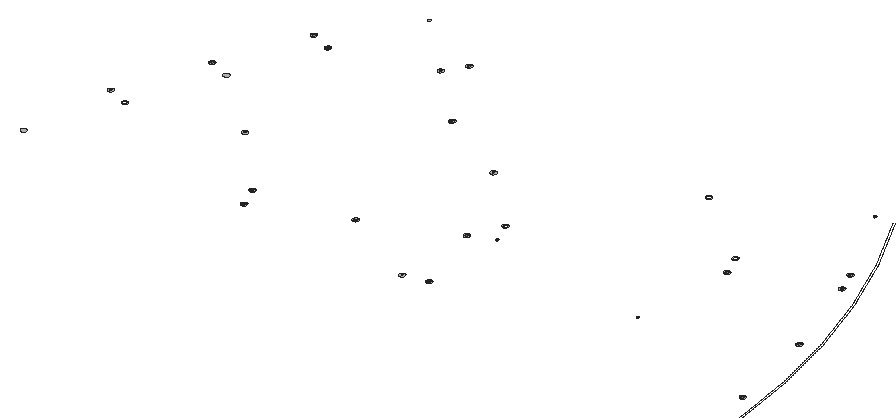
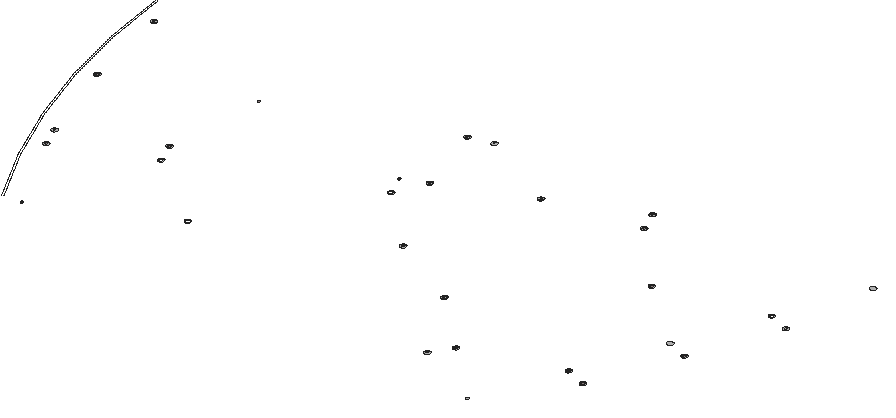
# SketchUp Ruby script. Lengths in inches.
U = 1.inch
M = Sketchup.active_model
def pt(a) = Geom::Point3d.new(a.map { |v| v * U })
def face(e, loops, mat)
  f = e.add_face(loops[0].map { |a| pt(a) })
  loops[1..].each { |l| e.add_face(l.map { |a| pt(a) }).erase! }
  f.material = f.back_material = mat if mat
  f
end
# faces: each face lists its corners as indices into pts; further lists are holes
def faces(e, pts, list, mat = nil) = list.each { |f| face(e, (f[0].is_a?(Array) ? f : [f]).map { |l| l.map { |i| pts[i] } }, mat) }
# xy, xz, yz: faces in a plane at the given z, y or x. An outline is a flat list of corners, or four numbers for a rectangle; further outlines are holes
def ring(l) = l.size == 4 ? [[l[0], l[1]], [l[2], l[1]], [l[2], l[3]], [l[0], l[3]]] : l.each_slice(2).to_a
def flat(e, list, mat, &to3) = list.each { |f| face(e, (f[0].is_a?(Array) ? f : [f]).map { |l| ring(l).map { |u, v| to3.(u, v) } }, mat) }
def xy(e, z, list, mat = nil) = flat(e, list, mat) { |x, y| [x, y, z] }
def xz(e, y, list, mat = nil) = flat(e, list, mat) { |x, z| [x, y, z] }
def yz(e, x, list, mat = nil) = flat(e, list, mat) { |y, z| [x, y, z] }
def lines(e, pts, list) = list.each { |a, b| e.add_line(pt(pts[a]), pt(pts[b])) }
# prism: a flat outline (further loops are holes) pulled along v
def prism(e, loops, v, mat = nil)
  f = face(e, loops, mat); d = Geom::Vector3d.new(v.map { |x| x * U })
  f.pushpull(f.normal.samedirection?(d) ? d.length : -d.length)
end
def box(e, o, s, mat = nil) = prism(e, [[o, [o[0] + s[0], o[1], o[2]], [o[0] + s[0], o[1] + s[1], o[2]], [o[0], o[1] + s[1], o[2]]]], [0, 0, s[2]], mat)
def at(x, y, z, deg = 0) = Geom::Transformation.translation(pt([x, y, z])) * Geom::Transformation.rotation(ORIGIN, Z_AXIS, deg.degrees)
def axes(o, x, y, z) = Geom::Transformation.new([*x, 0, *y, 0, *z, 0, *pt(o).to_a, 1])
def part(name) = M.definitions.add(name)
# library, detail: a bought-in or finely detailed component or shape, given as its bounding box
def library(name, o, s) = part(name).tap { |d| box(d.entities, o, s) }
def detail(e, o, s) = box(e.add_group.entities, o, s)
def put(e, d, t, mat = nil) = e.add_instance(d, t).tap { |i| i.material = mat if mat }
def group(e, t, mat = nil) = e.add_group.tap { |g| g.transformation = t; g.material = mat if mat }.entities
root = M.entities
M.materials.add("[Asphalt_Stamped_Brick]").color = [149, 133, 134]
M.materials.add("[Metal_Steel_Textured_White]").color = [191, 191, 191]
xy(root,3.625,[[165.183,166.325,165.178,166.327,165.174,166.33,165.171,166.335,165.169,166.339,165.168,166.345,165.169,166.35,165.171,166.355,165.174,166.359,165.178,166.362,165.183,166.364,165.188,166.365,165.193,166.364,165.198,166.362,165.202,166.359,165.205,166.355,165.207,166.35,165.208,166.345,165.207,166.339,165.205,166.335,165.202,166.33,165.198,166.327,165.193,166.325],[158.582,166.555,158.577,166.556,158.572,166.558,158.568,166.561,158.564,166.565,158.5625,166.57,158.562,166.575,158.5625,166.581,158.564,166.585,158.568,166.59,158.572,166.593,158.577,166.595,158.587,166.595,158.592,166.593,158.596,166.59,158.599,166.585,158.601,166.581,158.602,166.575,158.601,166.57,158.599,166.565,158.596,166.561,158.592,166.558,158.587,166.556],[175.826,166.647,175.821,166.648,175.816,166.65,175.812,166.653,175.809,166.657,175.807,166.662,175.806,166.667,175.807,166.672,175.809,166.677,175.812,166.681,175.816,166.685,175.821,166.687,175.831,166.687,175.836,166.685,175.84,166.681,175.843,166.677,175.845,166.672,175.846,166.667,175.845,166.662,175.843,166.657,175.84,166.653,175.836,166.65,175.831,166.648],[158.276,167.293,158.271,167.294,158.266,167.296,158.262,167.299,158.259,167.303,158.257,167.308,158.256,167.313,158.257,167.318,158.259,167.323,158.262,167.327,158.266,167.33,158.271,167.332,158.276,167.333,158.281,167.332,158.286,167.33,158.29,167.327,158.294,167.323,158.296,167.318,158.296,167.308,158.294,167.303,158.29,167.299,158.286,167.296,158.281,167.294],[170.838,168.324,170.833,168.326,170.829,168.329,170.826,168.334,170.824,168.338,170.823,168.344,170.824,168.349,170.826,168.354,170.829,168.358,170.833,168.361,170.838,168.363,170.843,168.364,170.849,168.363,170.853,168.361,170.858,168.358,170.861,168.354,170.863,168.349,170.863,168.338,170.861,168.334,170.858,168.329,170.853,168.326,170.849,168.324],
  [164.389,168.961,164.384,168.962,164.379,168.964,164.375,168.967,164.372,168.971,164.37,168.976,164.369,168.981,164.37,168.986,164.372,168.991,164.375,168.995,164.379,168.998,164.384,169,164.389,169.001,164.395,169,164.399,168.998,164.403,168.995,164.407,168.991,164.409,168.986,164.409,168.976,164.407,168.971,164.403,168.967,164.399,168.964,164.395,168.962],[165.183,169.292,165.178,169.294,165.174,169.298,165.171,169.302,165.169,169.307,165.168,169.312,165.169,169.317,165.171,169.322,165.174,169.326,165.178,169.329,165.183,169.331,165.188,169.332,165.193,169.331,165.198,169.329,165.202,169.326,165.205,169.322,165.207,169.317,165.208,169.312,165.207,169.307,165.205,169.302,165.202,169.298,165.198,169.294,165.193,169.292],[156.122,169.662,156.117,169.663,156.112,169.665,156.108,169.668,156.105,169.672,156.103,169.677,156.102,169.682,156.103,169.687,156.105,169.692,156.108,169.696,156.112,169.699,156.117,169.701,156.122,169.702,156.128,169.701,156.132,169.699,156.136,169.696,156.14,169.692,156.142,169.687,156.142,169.677,156.14,169.672,156.136,169.668,156.132,169.665,156.128,169.663],[175.208,169.885,175.202,169.886,175.198,169.888,175.193,169.891,175.19,169.895,175.188,169.9,175.1875,169.905,175.188,169.91,175.19,169.915,175.193,169.919,175.198,169.922,175.202,169.924,175.208,169.925,175.213,169.924,175.218,169.922,175.222,169.919,175.225,169.915,175.227,169.91,175.227,169.9,175.225,169.895,175.222,169.891,175.218,169.888,175.213,169.886],[171.188,171.777,171.183,171.778,171.178,171.78,171.174,171.783,171.17,171.787,171.168,171.792,171.168,171.802,171.17,171.807,171.174,171.811,171.178,171.814,171.183,171.816,171.188,171.817,171.193,171.816,171.198,171.814,171.202,171.811,171.205,171.807,171.207,171.802,171.208,171.797,171.207,171.792,171.205,171.787,171.202,171.783,171.198,171.78,171.193,171.778],
  [153.016,172.121,153.011,172.122,153.006,172.124,153.002,172.127,152.999,172.131,152.997,172.136,152.996,172.141,152.997,172.146,152.999,172.151,153.002,172.155,153.006,172.159,153.011,172.161,153.021,172.161,153.026,172.159,153.03,172.155,153.033,172.151,153.035,172.146,153.036,172.141,153.035,172.136,153.033,172.131,153.03,172.127,153.026,172.124,153.021,172.122],[162.779,172.128,162.774,172.13,162.77,172.133,162.767,172.138,162.765,172.142,162.764,172.147,162.765,172.153,162.767,172.157,162.77,172.162,162.774,172.165,162.779,172.167,162.789,172.167,162.794,172.165,162.798,172.162,162.801,172.157,162.803,172.153,162.804,172.147,162.803,172.142,162.801,172.138,162.798,172.133,162.794,172.13,162.789,172.128],[174.183,173.02,174.178,173.022,174.174,173.025,174.17,173.03,174.168,173.034,174.168,173.045,174.17,173.05,174.174,173.054,174.178,173.057,174.183,173.059,174.1875,173.06,174.193,173.059,174.198,173.057,174.202,173.054,174.205,173.05,174.207,173.045,174.208,173.04,174.207,173.034,174.205,173.03,174.202,173.025,174.198,173.022,174.193,173.02],[173.882,173.757,173.877,173.758,173.872,173.76,173.868,173.763,173.865,173.767,173.863,173.772,173.862,173.777,173.863,173.782,173.865,173.787,173.868,173.791,173.872,173.795,173.877,173.797,173.887,173.797,173.892,173.795,173.896,173.791,173.899,173.787,173.901,173.782,173.902,173.777,173.901,173.772,173.899,173.767,173.896,173.763,173.892,173.76,173.887,173.758],[154.951,174.72,154.946,174.722,154.942,174.725,154.939,174.73,154.937,174.734,154.936,174.74,154.937,174.745,154.939,174.75,154.942,174.754,154.946,174.757,154.951,174.759,154.956,174.76,154.962,174.759,154.966,174.757,154.97,174.754,154.974,174.75,154.976,174.745,154.976,174.734,154.974,174.73,154.97,174.725,154.966,174.722,154.962,174.72],
  [154.219,175.025,154.214,175.026,154.209,175.028,154.205,175.031,154.201,175.035,154.199,175.04,154.199,175.05,154.201,175.055,154.205,175.059,154.209,175.0625,154.214,175.064,154.219,175.065,154.224,175.064,154.229,175.0625,154.233,175.059,154.236,175.055,154.238,175.05,154.239,175.045,154.238,175.04,154.236,175.035,154.233,175.031,154.229,175.028,154.224,175.026],[158.583,176.324,158.578,176.326,158.574,176.33,158.571,176.334,158.569,176.339,158.568,176.344,158.569,176.349,158.571,176.354,158.574,176.358,158.578,176.361,158.583,176.363,158.588,176.364,158.593,176.363,158.598,176.361,158.602,176.358,158.605,176.354,158.607,176.349,158.608,176.344,158.607,176.339,158.605,176.334,158.602,176.33,158.598,176.326,158.593,176.324],[172.387,176.695,172.382,176.696,172.377,176.698,172.373,176.701,172.37,176.705,172.368,176.71,172.367,176.715,172.368,176.72,172.37,176.725,172.373,176.729,172.377,176.732,172.382,176.734,172.387,176.735,172.392,176.734,172.397,176.732,172.401,176.729,172.404,176.725,172.406,176.72,172.407,176.715,172.406,176.71,172.404,176.705,172.401,176.701,172.397,176.698,172.392,176.696]],"[Asphalt_Stamped_Brick]")
xy(root,3.625,[[[151.348,165.94,151.325,165.943,151.304,165.952,151.286,165.966,151.272,165.984,151.263,166.005,151.26,166.028,151.263,166.051,151.272,166.072,151.286,166.09,151.304,166.104,151.325,166.113,151.348,166.116,151.371,166.113,151.392,166.104,151.41,166.09,151.424,166.072,151.433,166.051,151.436,166.028,151.433,166.005,151.424,165.984,151.41,165.966,151.392,165.952,151.371,165.943],[151.348,165.992,151.357,165.993,151.366,165.996,151.374,166.002,151.38,166.01,151.383,166.019,151.385,166.028,151.383,166.038,151.38,166.046,151.374,166.054,151.366,166.06,151.357,166.064,151.348,166.065,151.339,166.064,151.33,166.06,151.322,166.054,151.316,166.046,151.3125,166.038,151.311,166.028,151.3125,166.019,151.316,166.01,151.322,166.002,151.33,165.996,151.339,165.993]],[[164.389,166.091,164.367,166.094,164.345,166.103,164.327,166.117,164.313,166.135,164.304,166.156,164.301,166.179,164.304,166.202,164.313,166.223,164.327,166.241,164.345,166.255,164.367,166.264,164.389,166.267,164.412,166.264,164.433,166.255,164.452,166.241,164.466,166.223,164.474,166.202,164.477,166.179,164.474,166.156,164.466,166.135,164.452,166.117,164.433,166.103,164.412,166.094],[164.389,166.143,164.399,166.144,164.408,166.148,164.415,166.153,164.421,166.161,164.425,166.17,164.426,166.179,164.425,166.189,164.421,166.198,164.415,166.205,164.408,166.211,164.399,166.215,164.389,166.216,164.38,166.215,164.371,166.211,164.363,166.205,164.358,166.198,164.354,166.189,164.353,166.179,164.354,166.17,164.358,166.161,164.363,166.153,164.371,166.148,164.38,166.144]],[164.389,166.159,164.384,166.16,164.379,166.162,164.375,166.165,164.372,166.169,164.37,166.174,164.369,166.179,164.37,166.184,164.372,166.189,164.375,166.193,164.379,166.197,164.389,166.199,164.395,166.198,164.399,166.197,164.407,166.189,164.409,166.184,164.409,166.174,164.407,166.169,164.403,166.165,164.399,166.162,164.395,166.16],[[165.188,166.256,165.165,166.259,165.143,166.268,165.125,166.282,165.111,166.3,165.102,166.322,165.099,166.345,165.102,166.368,165.111,166.389,165.125,166.407,165.143,166.422,165.165,166.43,165.188,166.433,165.211,166.43,165.232,166.422,165.251,166.407,165.265,166.389,165.274,166.368,165.277,166.345,165.274,166.322,165.265,166.3,165.251,166.282,165.232,166.268,165.211,166.259],[165.188,166.257,165.211,166.26,165.232,166.268,165.25,166.282,165.264,166.301,165.273,166.322,165.276,166.345,165.273,166.367,165.264,166.389,165.25,166.407,165.232,166.421,165.211,166.43,165.188,166.433,165.165,166.43,165.144,166.421,165.126,166.407,165.112,166.389,165.103,166.367,165.1,166.345,165.103,166.322,165.112,166.301,165.126,166.282,165.144,166.268,165.165,166.26]],[[165.188,166.308,165.178,166.309,165.169,166.313,165.162,166.319,165.156,166.326,165.152,166.335,165.151,166.345,165.152,166.354,165.156,166.363,165.162,166.37,165.169,166.376,165.178,166.38,165.188,166.381,165.197,166.38,165.206,166.376,165.214,166.37,165.219,166.363,165.223,166.354,165.224,166.345,165.223,166.335,165.219,166.326,165.214,166.319,165.206,166.313,165.197,166.309],[165.183,166.325,165.193,166.325,165.198,166.327,165.202,166.33,165.205,166.335,165.207,166.339,165.208,166.345,165.207,166.35,165.205,166.355,165.202,166.359,165.198,166.362,165.193,166.364,165.188,166.365,165.183,166.364,165.178,166.362,165.174,166.359,165.171,166.355,165.169,166.35,165.168,166.345,165.169,166.339,165.171,166.335,165.174,166.33,165.178,166.327]],
  [[158.582,166.487,158.559,166.49,158.537,166.498,158.519,166.513,158.505,166.531,158.496,166.552,158.493,166.575,158.496,166.598,158.505,166.62,158.519,166.638,158.537,166.652,158.559,166.661,158.582,166.664,158.605,166.661,158.626,166.652,158.645,166.638,158.659,166.62,158.668,166.598,158.671,166.575,158.668,166.552,158.659,166.531,158.645,166.513,158.626,166.498,158.605,166.49],[158.582,166.488,158.605,166.491,158.626,166.499,158.644,166.513,158.658,166.531,158.667,166.553,158.67,166.575,158.667,166.598,158.658,166.619,158.644,166.638,158.626,166.652,158.605,166.66,158.582,166.663,158.559,166.66,158.538,166.652,158.52,166.638,158.506,166.619,158.497,166.598,158.494,166.575,158.497,166.553,158.506,166.531,158.52,166.513,158.538,166.499,158.559,166.491]],[[158.582,166.488,158.559,166.491,158.538,166.499,158.52,166.513,158.506,166.531,158.497,166.553,158.494,166.575,158.497,166.598,158.506,166.619,158.52,166.638,158.538,166.652,158.559,166.66,158.582,166.663,158.605,166.66,158.626,166.652,158.644,166.638,158.658,166.619,158.667,166.598,158.67,166.575,158.667,166.553,158.658,166.531,158.644,166.513,158.626,166.499,158.605,166.491],[158.582,166.539,158.591,166.54,158.6,166.544,158.608,166.55,158.613,166.557,158.617,166.566,158.618,166.575,158.617,166.585,158.613,166.594,158.608,166.601,158.6,166.607,158.591,166.611,158.582,166.612,158.572,166.611,158.563,166.607,158.556,166.601,158.55,166.594,158.546,166.585,158.545,166.575,158.546,166.566,158.55,166.557,158.556,166.55,158.563,166.544,158.572,166.54]],[[158.582,166.539,158.572,166.54,158.563,166.544,158.556,166.55,158.55,166.557,158.546,166.566,158.545,166.575,158.546,166.585,158.55,166.594,158.556,166.601,158.563,166.607,158.572,166.611,158.582,166.612,158.591,166.611,158.6,166.607,158.608,166.601,158.613,166.594,158.617,166.585,158.618,166.575,158.617,166.566,158.613,166.557,158.608,166.55,158.6,166.544,158.591,166.54],[158.582,166.555,158.587,166.556,158.592,166.558,158.596,166.561,158.599,166.565,158.601,166.57,158.602,166.575,158.601,166.581,158.599,166.585,158.596,166.59,158.592,166.593,158.587,166.595,158.577,166.595,158.572,166.593,158.568,166.59,158.564,166.585,158.5625,166.581,158.562,166.575,158.5625,166.57,158.564,166.565,158.568,166.561,158.572,166.558,158.577,166.556]],[[175.826,166.578,175.803,166.581,175.782,166.59,175.763,166.604,175.749,166.623,175.74,166.644,175.737,166.667,175.74,166.69,175.749,166.712,175.763,166.73,175.782,166.744,175.803,166.753,175.826,166.756,175.849,166.753,175.87,166.744,175.889,166.73,175.903,166.712,175.912,166.69,175.915,166.667,175.912,166.644,175.903,166.623,175.889,166.604,175.87,166.59,175.849,166.581],[175.826,166.579,175.849,166.582,175.87,166.591,175.888,166.605,175.902,166.623,175.911,166.644,175.914,166.667,175.911,166.69,175.902,166.711,175.888,166.729,175.87,166.743,175.849,166.752,175.826,166.755,175.803,166.752,175.782,166.743,175.764,166.729,175.75,166.711,175.741,166.69,175.738,166.667,175.741,166.644,175.75,166.623,175.764,166.605,175.782,166.591,175.803,166.582]],[[175.826,166.579,175.803,166.582,175.782,166.591,175.764,166.605,175.75,166.623,175.741,166.644,175.738,166.667,175.741,166.69,175.75,166.711,175.764,166.729,175.782,166.743,175.803,166.752,175.826,166.755,175.849,166.752,175.87,166.743,175.888,166.729,175.902,166.711,175.911,166.69,175.914,166.667,175.911,166.644,175.902,166.623,175.888,166.605,175.87,166.591,175.849,166.582],[175.826,166.631,175.835,166.632,175.844,166.636,175.852,166.641,175.858,166.649,175.861,166.658,175.863,166.667,175.861,166.677,175.858,166.686,175.852,166.693,175.844,166.699,175.835,166.703,175.826,166.704,175.817,166.703,175.808,166.699,175.8,166.693,175.794,166.686,175.791,166.677,175.789,166.667,175.791,166.658,175.794,166.649,175.8,166.641,175.808,166.636,175.817,166.632]],
  [[175.826,166.631,175.817,166.632,175.808,166.636,175.8,166.641,175.794,166.649,175.791,166.658,175.789,166.667,175.791,166.677,175.794,166.686,175.8,166.693,175.808,166.699,175.817,166.703,175.826,166.704,175.835,166.703,175.844,166.699,175.852,166.693,175.858,166.686,175.861,166.677,175.863,166.667,175.861,166.658,175.858,166.649,175.852,166.641,175.844,166.636,175.835,166.632],[175.826,166.647,175.831,166.648,175.836,166.65,175.84,166.653,175.843,166.657,175.845,166.662,175.846,166.667,175.845,166.672,175.843,166.677,175.84,166.681,175.836,166.685,175.831,166.687,175.821,166.687,175.816,166.685,175.812,166.681,175.809,166.677,175.807,166.672,175.806,166.667,175.807,166.662,175.809,166.657,175.812,166.653,175.816,166.65,175.821,166.648]],[[158.276,167.224,158.253,167.227,158.232,167.236,158.213,167.25,158.199,167.269,158.19,167.29,158.1875,167.313,158.19,167.336,158.199,167.358,158.213,167.376,158.232,167.39,158.253,167.399,158.276,167.402,158.299,167.399,158.321,167.39,158.339,167.376,158.353,167.358,158.362,167.336,158.365,167.313,158.362,167.29,158.353,167.269,158.339,167.25,158.321,167.236,158.299,167.227],[158.276,167.225,158.299,167.228,158.32,167.237,158.338,167.251,158.352,167.269,158.361,167.29,158.364,167.313,158.361,167.336,158.352,167.357,158.338,167.375,158.32,167.389,158.299,167.398,158.276,167.401,158.253,167.398,158.232,167.389,158.214,167.375,158.2,167.357,158.191,167.336,158.188,167.313,158.191,167.29,158.2,167.269,158.214,167.251,158.232,167.237,158.253,167.228]],[[158.276,167.225,158.253,167.228,158.232,167.237,158.214,167.251,158.2,167.269,158.191,167.29,158.188,167.313,158.191,167.336,158.2,167.357,158.214,167.375,158.232,167.389,158.253,167.398,158.276,167.401,158.299,167.398,158.32,167.389,158.338,167.375,158.352,167.357,158.361,167.336,158.364,167.313,158.361,167.29,158.352,167.269,158.338,167.251,158.32,167.237,158.299,167.228],[158.276,167.276,158.286,167.278,158.295,167.281,158.302,167.287,158.308,167.295,158.312,167.304,158.313,167.313,158.312,167.323,158.308,167.331,158.302,167.339,158.295,167.345,158.286,167.348,158.276,167.35,158.267,167.348,158.258,167.345,158.25,167.339,158.245,167.331,158.241,167.323,158.24,167.313,158.241,167.304,158.245,167.295,158.25,167.287,158.258,167.281,158.267,167.278]],[[158.276,167.276,158.267,167.278,158.258,167.281,158.25,167.287,158.245,167.295,158.241,167.304,158.24,167.313,158.241,167.323,158.245,167.331,158.25,167.339,158.258,167.345,158.267,167.348,158.276,167.35,158.286,167.348,158.295,167.345,158.302,167.339,158.308,167.331,158.312,167.323,158.313,167.313,158.312,167.304,158.308,167.295,158.302,167.287,158.295,167.281,158.286,167.278],[158.276,167.293,158.281,167.294,158.286,167.296,158.29,167.299,158.294,167.303,158.296,167.308,158.296,167.318,158.294,167.323,158.29,167.327,158.286,167.33,158.281,167.332,158.276,167.333,158.271,167.332,158.266,167.33,158.262,167.327,158.259,167.323,158.257,167.318,158.256,167.313,158.257,167.308,158.259,167.303,158.262,167.299,158.266,167.296,158.271,167.294]],[[161.486,167.689,161.463,167.692,161.441,167.701,161.423,167.715,161.409,167.734,161.4,167.755,161.397,167.778,161.4,167.801,161.409,167.823,161.423,167.841,161.441,167.855,161.463,167.864,161.486,167.867,161.509,167.864,161.53,167.855,161.548,167.841,161.5625,167.823,161.571,167.801,161.574,167.778,161.571,167.755,161.5625,167.734,161.548,167.715,161.53,167.701,161.509,167.692],[161.486,167.69,161.508,167.693,161.53,167.702,161.548,167.716,161.562,167.734,161.57,167.755,161.573,167.778,161.57,167.801,161.562,167.822,161.548,167.84,161.53,167.854,161.508,167.863,161.486,167.866,161.463,167.863,161.442,167.854,161.423,167.84,161.409,167.822,161.401,167.801,161.398,167.778,161.401,167.755,161.409,167.734,161.423,167.716,161.442,167.702,161.463,167.693]],
  [[161.486,167.69,161.463,167.693,161.442,167.702,161.423,167.716,161.409,167.734,161.401,167.755,161.398,167.778,161.401,167.801,161.409,167.822,161.423,167.84,161.442,167.854,161.463,167.863,161.486,167.866,161.508,167.863,161.53,167.854,161.548,167.84,161.562,167.822,161.57,167.801,161.573,167.778,161.57,167.755,161.562,167.734,161.548,167.716,161.53,167.702,161.508,167.693],[161.486,167.742,161.495,167.743,161.504,167.747,161.511,167.752,161.517,167.76,161.521,167.769,161.522,167.778,161.521,167.788,161.517,167.797,161.511,167.804,161.504,167.81,161.495,167.814,161.486,167.815,161.476,167.814,161.467,167.81,161.46,167.804,161.454,167.797,161.45,167.788,161.449,167.778,161.45,167.769,161.454,167.76,161.46,167.752,161.467,167.747,161.476,167.743]],[161.486,167.758,161.48,167.759,161.476,167.761,161.471,167.764,161.468,167.768,161.466,167.773,161.466,167.783,161.468,167.788,161.471,167.792,161.476,167.796,161.48,167.798,161.491,167.798,161.496,167.796,161.5,167.792,161.503,167.788,161.505,167.783,161.506,167.778,161.505,167.773,161.503,167.768,161.5,167.764,161.496,167.761,161.491,167.759],[[170.843,168.307,170.834,168.308,170.825,168.312,170.818,168.318,170.812,168.325,170.808,168.334,170.807,168.344,170.808,168.353,170.812,168.362,170.818,168.369,170.825,168.375,170.834,168.379,170.843,168.38,170.853,168.379,170.862,168.375,170.869,168.369,170.875,168.362,170.879,168.353,170.88,168.344,170.879,168.334,170.875,168.325,170.869,168.318,170.862,168.312,170.853,168.308],[170.838,168.324,170.849,168.324,170.853,168.326,170.858,168.329,170.861,168.334,170.863,168.338,170.863,168.349,170.861,168.354,170.858,168.358,170.853,168.361,170.849,168.363,170.843,168.364,170.838,168.363,170.833,168.361,170.829,168.358,170.826,168.354,170.824,168.349,170.823,168.344,170.824,168.338,170.826,168.334,170.829,168.329,170.833,168.326]],[[152.551,168.843,152.528,168.846,152.506,168.855,152.488,168.869,152.474,168.888,152.465,168.909,152.462,168.932,152.465,168.955,152.474,168.976,152.488,168.995,152.506,169.009,152.528,169.018,152.551,169.021,152.574,169.018,152.595,169.009,152.614,168.995,152.628,168.976,152.637,168.955,152.64,168.932,152.637,168.909,152.628,168.888,152.614,168.869,152.595,168.855,152.574,168.846],[152.551,168.844,152.574,168.847,152.595,168.856,152.613,168.87,152.627,168.888,152.636,168.909,152.639,168.932,152.636,168.955,152.627,168.976,152.613,168.994,152.595,169.008,152.574,169.017,152.551,169.02,152.528,169.017,152.507,169.008,152.489,168.994,152.475,168.976,152.466,168.955,152.463,168.932,152.466,168.909,152.475,168.888,152.489,168.87,152.507,168.856,152.528,168.847]],[[164.389,168.892,164.366,168.895,164.345,168.904,164.327,168.918,164.3125,168.937,164.303,168.958,164.3,168.981,164.303,169.004,164.3125,169.025,164.327,169.044,164.345,169.058,164.366,169.067,164.389,169.07,164.412,169.067,164.434,169.058,164.452,169.044,164.466,169.025,164.475,169.004,164.478,168.981,164.475,168.958,164.466,168.937,164.452,168.918,164.434,168.904,164.412,168.895],[164.389,168.893,164.412,168.896,164.433,168.905,164.452,168.919,164.466,168.937,164.474,168.958,164.477,168.981,164.474,169.004,164.466,169.025,164.452,169.043,164.433,169.057,164.412,169.066,164.389,169.069,164.367,169.066,164.345,169.057,164.327,169.043,164.313,169.025,164.304,169.004,164.301,168.981,164.304,168.958,164.313,168.937,164.327,168.919,164.345,168.905,164.367,168.896]],
  [[164.389,168.893,164.367,168.896,164.345,168.905,164.327,168.919,164.313,168.937,164.304,168.958,164.301,168.981,164.304,169.004,164.313,169.025,164.327,169.043,164.345,169.057,164.367,169.066,164.389,169.069,164.412,169.066,164.433,169.057,164.452,169.043,164.466,169.025,164.474,169.004,164.477,168.981,164.474,168.958,164.466,168.937,164.452,168.919,164.433,168.905,164.412,168.896],[164.389,168.944,164.399,168.946,164.408,168.949,164.415,168.955,164.421,168.963,164.425,168.972,164.426,168.981,164.425,168.99,164.421,168.999,164.415,169.007,164.408,169.013,164.399,169.016,164.389,169.018,164.38,169.016,164.371,169.013,164.363,169.007,164.358,168.999,164.354,168.99,164.353,168.981,164.354,168.972,164.358,168.963,164.363,168.955,164.371,168.949,164.38,168.946]],[[164.389,168.944,164.38,168.946,164.371,168.949,164.363,168.955,164.358,168.963,164.354,168.972,164.353,168.981,164.354,168.99,164.358,168.999,164.363,169.007,164.371,169.013,164.38,169.016,164.389,169.018,164.399,169.016,164.408,169.013,164.415,169.007,164.421,168.999,164.425,168.99,164.426,168.981,164.425,168.972,164.421,168.963,164.415,168.955,164.408,168.949,164.399,168.946],[164.389,168.961,164.395,168.962,164.399,168.964,164.403,168.967,164.407,168.971,164.409,168.976,164.409,168.986,164.407,168.991,164.403,168.995,164.399,168.998,164.395,169,164.389,169.001,164.384,169,164.379,168.998,164.375,168.995,164.372,168.991,164.37,168.986,164.369,168.981,164.37,168.976,164.372,168.971,164.375,168.967,164.379,168.964,164.384,168.962]],[[151.813,169.15,151.79,169.153,151.769,169.161,151.751,169.175,151.737,169.194,151.728,169.215,151.725,169.238,151.728,169.26,151.737,169.281,151.751,169.3,151.769,169.314,151.79,169.322,151.813,169.325,151.836,169.322,151.857,169.314,151.875,169.3,151.889,169.281,151.898,169.26,151.901,169.238,151.898,169.215,151.889,169.194,151.875,169.175,151.857,169.161,151.836,169.153],[151.813,169.201,151.823,169.202,151.831,169.206,151.839,169.212,151.845,169.219,151.848,169.228,151.85,169.238,151.848,169.247,151.845,169.256,151.839,169.263,151.831,169.269,151.823,169.273,151.813,169.274,151.804,169.273,151.795,169.269,151.787,169.263,151.781,169.256,151.778,169.247,151.777,169.238,151.778,169.228,151.781,169.219,151.787,169.212,151.795,169.206,151.804,169.202]],[151.808,169.218,151.803,169.22,151.799,169.223,151.796,169.228,151.794,169.232,151.793,169.238,151.794,169.243,151.796,169.248,151.799,169.252,151.803,169.255,151.808,169.257,151.818,169.257,151.823,169.255,151.827,169.252,151.83,169.248,151.832,169.243,151.833,169.238,151.832,169.232,151.83,169.228,151.827,169.223,151.823,169.22,151.818,169.218],[[165.188,169.275,165.178,169.276,165.169,169.28,165.162,169.286,165.156,169.293,165.152,169.302,165.151,169.312,165.152,169.321,165.156,169.33,165.162,169.338,165.169,169.343,165.178,169.347,165.188,169.348,165.197,169.347,165.206,169.343,165.214,169.338,165.219,169.33,165.223,169.321,165.224,169.312,165.223,169.302,165.219,169.293,165.214,169.286,165.206,169.28,165.197,169.276],[165.183,169.292,165.193,169.292,165.198,169.294,165.202,169.298,165.205,169.302,165.207,169.307,165.208,169.312,165.207,169.317,165.205,169.322,165.202,169.326,165.198,169.329,165.193,169.331,165.188,169.332,165.183,169.331,165.178,169.329,165.174,169.326,165.171,169.322,165.169,169.317,165.168,169.312,165.169,169.307,165.171,169.302,165.174,169.298,165.178,169.294]],
  [[156.122,169.594,156.1,169.597,156.078,169.606,156.06,169.62,156.046,169.638,156.037,169.659,156.034,169.682,156.037,169.705,156.046,169.726,156.06,169.744,156.078,169.758,156.1,169.767,156.122,169.77,156.145,169.767,156.166,169.758,156.185,169.744,156.199,169.726,156.207,169.705,156.21,169.682,156.207,169.659,156.199,169.638,156.185,169.62,156.166,169.606,156.145,169.597],[156.122,169.645,156.132,169.647,156.141,169.65,156.148,169.656,156.154,169.664,156.158,169.672,156.159,169.682,156.158,169.691,156.154,169.7,156.148,169.708,156.141,169.714,156.132,169.717,156.122,169.718,156.113,169.717,156.104,169.714,156.096,169.708,156.091,169.7,156.087,169.691,156.086,169.682,156.087,169.672,156.091,169.664,156.096,169.656,156.104,169.65,156.113,169.647]],[[156.122,169.645,156.113,169.647,156.104,169.65,156.096,169.656,156.091,169.664,156.087,169.672,156.086,169.682,156.087,169.691,156.091,169.7,156.096,169.708,156.104,169.714,156.113,169.717,156.122,169.718,156.132,169.717,156.141,169.714,156.148,169.708,156.154,169.7,156.158,169.691,156.159,169.682,156.158,169.672,156.154,169.664,156.148,169.656,156.141,169.65,156.132,169.647],[156.122,169.662,156.128,169.663,156.132,169.665,156.136,169.668,156.14,169.672,156.142,169.677,156.142,169.687,156.14,169.692,156.136,169.696,156.132,169.699,156.128,169.701,156.122,169.702,156.117,169.701,156.112,169.699,156.108,169.696,156.105,169.692,156.103,169.687,156.102,169.682,156.103,169.677,156.105,169.672,156.108,169.668,156.112,169.665,156.117,169.663]],[[175.208,169.816,175.185,169.819,175.163,169.828,175.145,169.842,175.131,169.861,175.122,169.882,175.119,169.905,175.122,169.928,175.131,169.949,175.145,169.968,175.163,169.982,175.185,169.991,175.208,169.994,175.231,169.991,175.252,169.982,175.27,169.968,175.285,169.949,175.293,169.928,175.296,169.905,175.293,169.882,175.285,169.861,175.27,169.842,175.252,169.828,175.231,169.819],[175.208,169.817,175.23,169.82,175.252,169.829,175.27,169.843,175.284,169.861,175.292,169.882,175.295,169.905,175.292,169.928,175.284,169.949,175.27,169.967,175.252,169.981,175.23,169.99,175.208,169.993,175.185,169.99,175.164,169.981,175.145,169.967,175.131,169.949,175.123,169.928,175.12,169.905,175.123,169.882,175.131,169.861,175.145,169.843,175.164,169.829,175.185,169.82]],[[175.208,169.817,175.185,169.82,175.164,169.829,175.145,169.843,175.131,169.861,175.123,169.882,175.12,169.905,175.123,169.928,175.131,169.949,175.145,169.967,175.164,169.981,175.185,169.99,175.208,169.993,175.23,169.99,175.252,169.981,175.27,169.967,175.284,169.949,175.292,169.928,175.295,169.905,175.292,169.882,175.284,169.861,175.27,169.843,175.252,169.829,175.23,169.82],[175.208,169.868,175.217,169.87,175.226,169.873,175.233,169.879,175.239,169.887,175.243,169.896,175.244,169.905,175.243,169.914,175.239,169.923,175.233,169.931,175.226,169.937,175.217,169.94,175.208,169.942,175.198,169.94,175.189,169.937,175.182,169.931,175.176,169.923,175.172,169.914,175.171,169.905,175.172,169.896,175.176,169.887,175.182,169.879,175.189,169.873,175.198,169.87]],[[175.208,169.868,175.198,169.87,175.189,169.873,175.182,169.879,175.176,169.887,175.172,169.896,175.171,169.905,175.172,169.914,175.176,169.923,175.182,169.931,175.189,169.937,175.198,169.94,175.208,169.942,175.217,169.94,175.226,169.937,175.233,169.931,175.239,169.923,175.243,169.914,175.244,169.905,175.243,169.896,175.239,169.887,175.233,169.879,175.226,169.873,175.217,169.87],[175.208,169.885,175.213,169.886,175.218,169.888,175.222,169.891,175.225,169.895,175.227,169.9,175.227,169.91,175.225,169.915,175.222,169.919,175.218,169.922,175.213,169.924,175.208,169.925,175.202,169.924,175.198,169.922,175.193,169.919,175.19,169.915,175.188,169.91,175.1875,169.905,175.188,169.9,175.19,169.895,175.193,169.891,175.198,169.888,175.202,169.886]],
  [[164.882,169.961,164.859,169.964,164.838,169.972,164.819,169.987,164.805,170.005,164.796,170.026,164.793,170.049,164.796,170.072,164.805,170.094,164.819,170.112,164.838,170.126,164.859,170.135,164.882,170.138,164.905,170.135,164.927,170.126,164.945,170.112,164.959,170.094,164.968,170.072,164.971,170.049,164.968,170.026,164.959,170.005,164.945,169.987,164.927,169.972,164.905,169.964],[164.882,169.961,164.905,169.964,164.926,169.973,164.944,169.987,164.958,170.005,164.967,170.027,164.97,170.049,164.967,170.072,164.958,170.093,164.944,170.112,164.926,170.126,164.905,170.134,164.882,170.137,164.859,170.134,164.838,170.126,164.82,170.112,164.806,170.093,164.797,170.072,164.794,170.049,164.797,170.027,164.806,170.005,164.82,169.987,164.838,169.973,164.859,169.964]],[[171.188,171.708,171.165,171.711,171.143,171.72,171.125,171.734,171.111,171.753,171.102,171.774,171.099,171.797,171.102,171.82,171.111,171.841,171.125,171.86,171.143,171.874,171.165,171.883,171.188,171.886,171.211,171.883,171.232,171.874,171.251,171.86,171.265,171.841,171.274,171.82,171.277,171.797,171.274,171.774,171.265,171.753,171.251,171.734,171.232,171.72,171.211,171.711],[171.188,171.709,171.21,171.712,171.232,171.721,171.25,171.735,171.264,171.753,171.273,171.774,171.276,171.797,171.273,171.82,171.264,171.841,171.25,171.859,171.232,171.873,171.21,171.882,171.188,171.885,171.165,171.882,171.144,171.873,171.126,171.859,171.112,171.841,171.103,171.82,171.1,171.797,171.103,171.774,171.112,171.753,171.126,171.735,171.144,171.721,171.165,171.712]],[[153.754,171.748,153.731,171.751,153.71,171.76,153.691,171.774,153.677,171.792,153.669,171.813,153.666,171.836,153.669,171.859,153.677,171.88,153.691,171.898,153.71,171.912,153.731,171.921,153.754,171.924,153.776,171.921,153.798,171.912,153.816,171.898,153.83,171.88,153.838,171.859,153.841,171.836,153.838,171.813,153.83,171.792,153.816,171.774,153.798,171.76,153.776,171.751],[153.754,171.799,153.763,171.8,153.772,171.804,153.779,171.81,153.785,171.817,153.789,171.826,153.79,171.836,153.789,171.845,153.785,171.854,153.779,171.862,153.772,171.867,153.763,171.871,153.754,171.872,153.744,171.871,153.735,171.867,153.728,171.862,153.722,171.854,153.718,171.845,153.717,171.836,153.718,171.826,153.722,171.817,153.728,171.81,153.735,171.804,153.744,171.8]],[[171.188,171.76,171.178,171.762,171.169,171.765,171.162,171.771,171.156,171.779,171.152,171.788,171.151,171.797,171.152,171.806,171.156,171.815,171.162,171.823,171.169,171.829,171.178,171.832,171.188,171.834,171.197,171.832,171.206,171.829,171.214,171.823,171.219,171.815,171.223,171.806,171.224,171.797,171.223,171.788,171.219,171.779,171.214,171.771,171.206,171.765,171.197,171.762],[171.188,171.777,171.193,171.778,171.198,171.78,171.202,171.783,171.205,171.787,171.207,171.792,171.208,171.797,171.207,171.802,171.205,171.807,171.202,171.811,171.198,171.814,171.193,171.816,171.188,171.817,171.183,171.816,171.178,171.814,171.174,171.811,171.17,171.807,171.168,171.802,171.168,171.792,171.17,171.787,171.174,171.783,171.178,171.78,171.183,171.778]],[[153.016,172.052,152.993,172.055,152.971,172.064,152.953,172.078,152.939,172.097,152.93,172.118,152.927,172.141,152.93,172.164,152.939,172.186,152.953,172.204,152.971,172.218,152.993,172.227,153.016,172.23,153.039,172.227,153.06,172.218,153.079,172.204,153.093,172.186,153.102,172.164,153.105,172.141,153.102,172.118,153.093,172.097,153.079,172.078,153.06,172.064,153.039,172.055],[153.016,172.053,153.039,172.056,153.06,172.065,153.078,172.079,153.092,172.097,153.101,172.119,153.104,172.141,153.101,172.164,153.092,172.185,153.078,172.203,153.06,172.217,153.039,172.226,153.016,172.229,152.993,172.226,152.972,172.217,152.954,172.203,152.94,172.185,152.931,172.164,152.928,172.141,152.931,172.119,152.94,172.097,152.954,172.079,152.972,172.065,152.993,172.056]],
  [[153.016,172.053,152.993,172.056,152.972,172.065,152.954,172.079,152.94,172.097,152.931,172.119,152.928,172.141,152.931,172.164,152.94,172.185,152.954,172.203,152.972,172.217,152.993,172.226,153.016,172.229,153.039,172.226,153.06,172.217,153.078,172.203,153.092,172.185,153.101,172.164,153.104,172.141,153.101,172.119,153.092,172.097,153.078,172.079,153.06,172.065,153.039,172.056],[153.016,172.105,153.025,172.106,153.034,172.11,153.042,172.115,153.048,172.123,153.051,172.132,153.052,172.141,153.051,172.151,153.048,172.16,153.042,172.167,153.034,172.173,153.025,172.177,153.016,172.178,153.006,172.177,152.998,172.173,152.99,172.167,152.984,172.16,152.981,172.151,152.979,172.141,152.981,172.132,152.984,172.123,152.99,172.115,152.998,172.11,153.006,172.106]],[[162.784,172.06,162.761,172.0625,162.74,172.071,162.722,172.085,162.708,172.104,162.699,172.125,162.696,172.147,162.699,172.17,162.708,172.191,162.722,172.21,162.74,172.224,162.761,172.232,162.784,172.235,162.807,172.232,162.828,172.224,162.846,172.21,162.86,172.191,162.869,172.17,162.872,172.147,162.869,172.125,162.86,172.104,162.846,172.085,162.828,172.071,162.807,172.0625],[162.784,172.111,162.794,172.112,162.802,172.116,162.81,172.122,162.816,172.129,162.819,172.138,162.821,172.147,162.819,172.157,162.816,172.166,162.81,172.173,162.802,172.179,162.794,172.183,162.784,172.184,162.775,172.183,162.766,172.179,162.758,172.173,162.752,172.166,162.749,172.157,162.748,172.147,162.749,172.138,162.752,172.129,162.758,172.122,162.766,172.116,162.775,172.112]],[[153.016,172.105,153.006,172.106,152.998,172.11,152.99,172.115,152.984,172.123,152.981,172.132,152.979,172.141,152.981,172.151,152.984,172.16,152.99,172.167,152.998,172.173,153.006,172.177,153.016,172.178,153.025,172.177,153.034,172.173,153.042,172.167,153.048,172.16,153.051,172.151,153.052,172.141,153.051,172.132,153.048,172.123,153.042,172.115,153.034,172.11,153.025,172.106],[153.016,172.121,153.021,172.122,153.026,172.124,153.03,172.127,153.033,172.131,153.035,172.136,153.036,172.141,153.035,172.146,153.033,172.151,153.03,172.155,153.026,172.159,153.021,172.161,153.011,172.161,153.006,172.159,153.002,172.155,152.999,172.151,152.997,172.146,152.996,172.141,152.997,172.136,152.999,172.131,153.002,172.127,153.006,172.124,153.011,172.122]],[[162.784,172.111,162.775,172.112,162.766,172.116,162.758,172.122,162.752,172.129,162.749,172.138,162.748,172.147,162.749,172.157,162.752,172.166,162.758,172.173,162.766,172.179,162.775,172.183,162.784,172.184,162.794,172.183,162.802,172.179,162.81,172.173,162.816,172.166,162.819,172.157,162.821,172.147,162.819,172.138,162.816,172.129,162.81,172.122,162.802,172.116,162.794,172.112],[162.779,172.128,162.789,172.128,162.794,172.13,162.798,172.133,162.801,172.138,162.803,172.142,162.804,172.147,162.803,172.153,162.801,172.157,162.798,172.162,162.794,172.165,162.789,172.167,162.779,172.167,162.774,172.165,162.77,172.162,162.767,172.157,162.765,172.153,162.764,172.147,162.765,172.142,162.767,172.138,162.77,172.133,162.774,172.13]],[[170.882,172.446,170.859,172.449,170.838,172.458,170.819,172.472,170.805,172.49,170.796,172.512,170.793,172.535,170.796,172.558,170.805,172.579,170.819,172.597,170.838,172.612,170.859,172.62,170.882,172.624,170.905,172.62,170.927,172.612,170.945,172.597,170.959,172.579,170.968,172.558,170.971,172.535,170.968,172.512,170.959,172.49,170.945,172.472,170.927,172.458,170.905,172.449],[170.882,172.447,170.905,172.45,170.926,172.458,170.944,172.472,170.958,172.491,170.967,172.512,170.97,172.535,170.967,172.557,170.958,172.579,170.944,172.597,170.926,172.611,170.905,172.62,170.882,172.623,170.859,172.62,170.838,172.611,170.82,172.597,170.806,172.579,170.797,172.557,170.794,172.535,170.797,172.512,170.806,172.491,170.82,172.472,170.838,172.458,170.859,172.45]],
  [[174.1875,172.952,174.165,172.955,174.144,172.963,174.125,172.977,174.112,172.996,174.103,173.017,174.1,173.04,174.103,173.0625,174.112,173.084,174.125,173.102,174.144,173.116,174.165,173.125,174.1875,173.128,174.21,173.125,174.232,173.116,174.25,173.102,174.264,173.084,174.273,173.0625,174.276,173.04,174.273,173.017,174.264,172.996,174.25,172.977,174.232,172.963,174.21,172.955],[174.1875,173.003,174.197,173.004,174.206,173.008,174.214,173.014,174.219,173.021,174.223,173.03,174.224,173.04,174.223,173.049,174.219,173.058,174.214,173.065,174.206,173.071,174.197,173.075,174.1875,173.076,174.178,173.075,174.169,173.071,174.162,173.065,174.156,173.058,174.152,173.049,174.151,173.04,174.152,173.03,174.156,173.021,174.162,173.014,174.169,173.008,174.178,173.004]],[[174.1875,173.003,174.178,173.004,174.169,173.008,174.162,173.014,174.156,173.021,174.152,173.03,174.151,173.04,174.152,173.049,174.156,173.058,174.162,173.065,174.169,173.071,174.178,173.075,174.1875,173.076,174.197,173.075,174.206,173.071,174.214,173.065,174.219,173.058,174.223,173.049,174.224,173.04,174.223,173.03,174.219,173.021,174.214,173.014,174.206,173.008,174.197,173.004],[174.183,173.02,174.193,173.02,174.198,173.022,174.202,173.025,174.205,173.03,174.207,173.034,174.208,173.04,174.207,173.045,174.205,173.05,174.202,173.054,174.198,173.057,174.193,173.059,174.1875,173.06,174.183,173.059,174.178,173.057,174.174,173.054,174.17,173.05,174.168,173.045,174.168,173.034,174.17,173.03,174.174,173.025,174.178,173.022]],[[160.121,173.592,160.098,173.595,160.077,173.604,160.059,173.618,160.044,173.637,160.036,173.658,160.033,173.681,160.036,173.704,160.044,173.725,160.059,173.744,160.077,173.758,160.098,173.767,160.121,173.77,160.144,173.767,160.166,173.758,160.184,173.744,160.198,173.725,160.207,173.704,160.21,173.681,160.207,173.658,160.198,173.637,160.184,173.618,160.166,173.604,160.144,173.595],[160.121,173.593,160.144,173.596,160.165,173.605,160.184,173.619,160.198,173.637,160.206,173.658,160.209,173.681,160.206,173.704,160.198,173.725,160.184,173.743,160.165,173.757,160.144,173.766,160.121,173.769,160.099,173.766,160.078,173.757,160.059,173.743,160.045,173.725,160.037,173.704,160.034,173.681,160.037,173.658,160.045,173.637,160.059,173.619,160.078,173.605,160.099,173.596]],[[160.121,173.644,160.112,173.646,160.103,173.649,160.096,173.655,160.09,173.663,160.086,173.672,160.085,173.681,160.086,173.69,160.09,173.699,160.096,173.707,160.103,173.713,160.112,173.716,160.121,173.718,160.131,173.716,160.14,173.713,160.147,173.707,160.153,173.699,160.157,173.69,160.158,173.681,160.157,173.672,160.153,173.663,160.147,173.655,160.14,173.649,160.131,173.646],[160.121,173.661,160.127,173.662,160.131,173.664,160.136,173.667,160.139,173.671,160.141,173.676,160.141,173.686,160.139,173.691,160.136,173.695,160.131,173.698,160.127,173.7,160.121,173.701,160.116,173.7,160.111,173.698,160.107,173.695,160.104,173.691,160.102,173.686,160.102,173.676,160.104,173.671,160.107,173.667,160.111,173.664,160.116,173.662]],[160.121,173.661,160.116,173.662,160.111,173.664,160.107,173.667,160.104,173.671,160.102,173.676,160.102,173.686,160.104,173.691,160.107,173.695,160.111,173.698,160.116,173.7,160.121,173.701,160.127,173.7,160.131,173.698,160.136,173.695,160.139,173.691,160.141,173.686,160.141,173.676,160.139,173.671,160.136,173.667,160.131,173.664,160.127,173.662],
  [[173.882,173.689,173.859,173.692,173.838,173.701,173.82,173.715,173.806,173.733,173.797,173.755,173.794,173.777,173.797,173.8,173.806,173.821,173.82,173.839,173.838,173.853,173.859,173.862,173.882,173.865,173.905,173.862,173.926,173.853,173.944,173.839,173.958,173.821,173.967,173.8,173.97,173.777,173.967,173.755,173.958,173.733,173.944,173.715,173.926,173.701,173.905,173.692],[173.882,173.741,173.892,173.742,173.9,173.746,173.908,173.751,173.914,173.759,173.917,173.768,173.919,173.777,173.917,173.787,173.914,173.796,173.908,173.803,173.9,173.809,173.892,173.8125,173.882,173.814,173.873,173.8125,173.864,173.809,173.856,173.803,173.85,173.796,173.847,173.787,173.846,173.777,173.847,173.768,173.85,173.759,173.856,173.751,173.864,173.746,173.873,173.742]],[[173.882,173.741,173.873,173.742,173.864,173.746,173.856,173.751,173.85,173.759,173.847,173.768,173.846,173.777,173.847,173.787,173.85,173.796,173.856,173.803,173.864,173.809,173.873,173.8125,173.882,173.814,173.892,173.8125,173.9,173.809,173.908,173.803,173.914,173.796,173.917,173.787,173.919,173.777,173.917,173.768,173.914,173.759,173.908,173.751,173.9,173.746,173.892,173.742],[173.882,173.757,173.887,173.758,173.892,173.76,173.896,173.763,173.899,173.767,173.901,173.772,173.902,173.777,173.901,173.782,173.899,173.787,173.896,173.791,173.892,173.795,173.887,173.797,173.877,173.797,173.872,173.795,173.868,173.791,173.865,173.787,173.863,173.782,173.862,173.777,173.863,173.772,173.865,173.767,173.868,173.763,173.872,173.76,173.877,173.758]],[[168.197,174.644,168.174,174.647,168.152,174.656,168.134,174.67,168.12,174.689,168.111,174.71,168.108,174.733,168.111,174.756,168.12,174.778,168.134,174.796,168.152,174.81,168.174,174.819,168.197,174.822,168.22,174.819,168.241,174.81,168.26,174.796,168.274,174.778,168.283,174.756,168.286,174.733,168.283,174.71,168.274,174.689,168.26,174.67,168.241,174.656,168.22,174.647],[168.197,174.645,168.22,174.648,168.241,174.657,168.259,174.671,168.273,174.689,168.282,174.71,168.285,174.733,168.282,174.756,168.273,174.777,168.259,174.795,168.241,174.809,168.22,174.818,168.197,174.821,168.174,174.818,168.153,174.809,168.135,174.795,168.121,174.777,168.112,174.756,168.109,174.733,168.112,174.71,168.121,174.689,168.135,174.671,168.153,174.657,168.174,174.648]],[[154.956,174.651,154.933,174.654,154.912,174.663,154.893,174.677,154.879,174.695,154.87,174.717,154.867,174.74,154.87,174.763,154.879,174.784,154.893,174.802,154.912,174.817,154.933,174.825,154.956,174.828,154.979,174.825,155.001,174.817,155.019,174.802,155.033,174.784,155.042,174.763,155.045,174.74,155.042,174.717,155.033,174.695,155.019,174.677,155.001,174.663,154.979,174.654],[154.956,174.652,154.979,174.655,155,174.663,155.019,174.677,155.032,174.696,155.041,174.717,155.044,174.74,155.041,174.762,155.032,174.784,155.019,174.802,155,174.816,154.979,174.824,154.956,174.827,154.934,174.824,154.912,174.816,154.894,174.802,154.88,174.784,154.871,174.762,154.868,174.74,154.871,174.717,154.88,174.696,154.894,174.677,154.912,174.663,154.934,174.655]],[[154.956,174.652,154.934,174.655,154.912,174.663,154.894,174.677,154.88,174.696,154.871,174.717,154.868,174.74,154.871,174.762,154.88,174.784,154.894,174.802,154.912,174.816,154.934,174.824,154.956,174.827,154.979,174.824,155,174.816,155.019,174.802,155.032,174.784,155.041,174.762,155.044,174.74,155.041,174.717,155.032,174.696,155.019,174.677,155,174.663,154.979,174.655],[154.956,174.703,154.966,174.704,154.975,174.708,154.982,174.714,154.988,174.721,154.992,174.73,154.993,174.74,154.992,174.749,154.988,174.758,154.982,174.765,154.975,174.771,154.966,174.775,154.956,174.776,154.947,174.775,154.938,174.771,154.93,174.765,154.925,174.758,154.921,174.749,154.92,174.74,154.921,174.73,154.925,174.721,154.93,174.714,154.938,174.708,154.947,174.704]],
  [[154.956,174.703,154.947,174.704,154.938,174.708,154.93,174.714,154.925,174.721,154.921,174.73,154.92,174.74,154.921,174.749,154.925,174.758,154.93,174.765,154.938,174.771,154.947,174.775,154.956,174.776,154.966,174.775,154.975,174.771,154.982,174.765,154.988,174.758,154.992,174.749,154.993,174.74,154.992,174.73,154.988,174.721,154.982,174.714,154.975,174.708,154.966,174.704],[154.951,174.72,154.962,174.72,154.966,174.722,154.97,174.725,154.974,174.73,154.976,174.734,154.976,174.745,154.974,174.75,154.97,174.754,154.966,174.757,154.962,174.759,154.956,174.76,154.951,174.759,154.946,174.757,154.942,174.754,154.939,174.75,154.937,174.745,154.936,174.74,154.937,174.734,154.939,174.73,154.942,174.725,154.946,174.722]],[[154.219,174.956,154.196,174.959,154.174,174.968,154.156,174.982,154.142,175.001,154.133,175.022,154.13,175.045,154.133,175.068,154.142,175.09,154.156,175.108,154.174,175.122,154.196,175.131,154.219,175.134,154.242,175.131,154.263,175.122,154.282,175.108,154.296,175.09,154.305,175.068,154.308,175.045,154.305,175.022,154.296,175.001,154.282,174.982,154.263,174.968,154.242,174.959],[154.219,174.957,154.241,174.96,154.263,174.969,154.281,174.983,154.295,175.001,154.304,175.022,154.307,175.045,154.304,175.068,154.295,175.089,154.281,175.107,154.263,175.121,154.241,175.13,154.219,175.133,154.196,175.13,154.175,175.121,154.157,175.107,154.143,175.089,154.134,175.068,154.131,175.045,154.134,175.022,154.143,175.001,154.157,174.983,154.175,174.969,154.196,174.96]],[[154.219,174.957,154.196,174.96,154.175,174.969,154.157,174.983,154.143,175.001,154.134,175.022,154.131,175.045,154.134,175.068,154.143,175.089,154.157,175.107,154.175,175.121,154.196,175.13,154.219,175.133,154.241,175.13,154.263,175.121,154.281,175.107,154.295,175.089,154.304,175.068,154.307,175.045,154.304,175.022,154.295,175.001,154.281,174.983,154.263,174.969,154.241,174.96],[154.219,175.009,154.228,175.01,154.237,175.013,154.245,175.019,154.25,175.027,154.254,175.036,154.255,175.045,154.254,175.055,154.25,175.063,154.245,175.071,154.237,175.077,154.228,175.08,154.219,175.082,154.209,175.08,154.2,175.077,154.193,175.071,154.187,175.063,154.183,175.055,154.182,175.045,154.183,175.036,154.187,175.027,154.193,175.019,154.2,175.013,154.209,175.01]],[[154.219,175.009,154.209,175.01,154.2,175.013,154.193,175.019,154.187,175.027,154.183,175.036,154.182,175.045,154.183,175.055,154.187,175.063,154.193,175.071,154.2,175.077,154.209,175.08,154.219,175.082,154.228,175.08,154.237,175.077,154.245,175.071,154.25,175.063,154.254,175.055,154.255,175.045,154.254,175.036,154.25,175.027,154.245,175.019,154.237,175.013,154.228,175.01],[154.219,175.025,154.224,175.026,154.229,175.028,154.233,175.031,154.236,175.035,154.238,175.04,154.239,175.045,154.238,175.05,154.236,175.055,154.233,175.059,154.229,175.0625,154.224,175.064,154.219,175.065,154.214,175.064,154.209,175.0625,154.205,175.059,154.201,175.055,154.199,175.05,154.199,175.04,154.201,175.035,154.205,175.031,154.209,175.028,154.214,175.026]],[[158.14,175.573,158.117,175.576,158.096,175.585,158.077,175.599,158.063,175.618,158.054,175.639,158.051,175.662,158.054,175.685,158.063,175.707,158.077,175.725,158.096,175.739,158.117,175.748,158.14,175.751,158.163,175.748,158.185,175.739,158.203,175.725,158.217,175.707,158.226,175.685,158.229,175.662,158.226,175.639,158.217,175.618,158.203,175.599,158.185,175.585,158.163,175.576],[158.14,175.574,158.163,175.577,158.184,175.586,158.202,175.6,158.216,175.618,158.225,175.639,158.228,175.662,158.225,175.685,158.216,175.706,158.202,175.724,158.184,175.738,158.163,175.747,158.14,175.75,158.118,175.747,158.096,175.738,158.078,175.724,158.064,175.706,158.055,175.685,158.052,175.662,158.055,175.639,158.064,175.618,158.078,175.6,158.096,175.586,158.118,175.577]],
  [[158.14,175.574,158.118,175.577,158.096,175.586,158.078,175.6,158.064,175.618,158.055,175.639,158.052,175.662,158.055,175.685,158.064,175.706,158.078,175.724,158.096,175.738,158.118,175.747,158.14,175.75,158.163,175.747,158.184,175.738,158.202,175.724,158.216,175.706,158.225,175.685,158.228,175.662,158.225,175.639,158.216,175.618,158.202,175.6,158.184,175.586,158.163,175.577],[158.14,175.626,158.15,175.627,158.159,175.63,158.166,175.636,158.172,175.644,158.176,175.653,158.177,175.662,158.176,175.672,158.172,175.68,158.166,175.688,158.159,175.694,158.15,175.698,158.14,175.699,158.131,175.698,158.122,175.694,158.114,175.688,158.109,175.68,158.105,175.672,158.104,175.662,158.105,175.653,158.109,175.644,158.114,175.636,158.122,175.63,158.131,175.627]],[[158.14,175.626,158.131,175.627,158.122,175.63,158.114,175.636,158.109,175.644,158.105,175.653,158.104,175.662,158.105,175.672,158.109,175.68,158.114,175.688,158.122,175.694,158.131,175.698,158.14,175.699,158.15,175.698,158.159,175.694,158.166,175.688,158.172,175.68,158.176,175.672,158.177,175.662,158.176,175.653,158.172,175.644,158.166,175.636,158.159,175.63,158.15,175.627],[158.14,175.642,158.145,175.643,158.15,175.645,158.154,175.648,158.158,175.652,158.16,175.657,158.16,175.667,158.158,175.672,158.154,175.676,158.15,175.679,158.145,175.681,158.14,175.682,158.135,175.681,158.13,175.679,158.126,175.676,158.123,175.672,158.121,175.667,158.12,175.662,158.121,175.657,158.123,175.652,158.126,175.648,158.13,175.645,158.135,175.643]],[158.14,175.642,158.135,175.643,158.13,175.645,158.126,175.648,158.123,175.652,158.121,175.657,158.12,175.662,158.121,175.667,158.123,175.672,158.126,175.676,158.13,175.679,158.135,175.681,158.14,175.682,158.145,175.681,158.15,175.679,158.154,175.676,158.158,175.672,158.16,175.667,158.16,175.657,158.158,175.652,158.154,175.648,158.15,175.645,158.145,175.643],[[158.588,176.256,158.565,176.259,158.544,176.268,158.526,176.282,158.512,176.3,158.503,176.321,158.5,176.344,158.503,176.366,158.512,176.388,158.526,176.406,158.544,176.42,158.565,176.429,158.588,176.432,158.611,176.429,158.632,176.42,158.65,176.406,158.664,176.388,158.673,176.366,158.676,176.344,158.673,176.321,158.664,176.3,158.65,176.282,158.632,176.268,158.611,176.259],[158.588,176.307,158.597,176.308,158.606,176.312,158.614,176.318,158.62,176.325,158.623,176.334,158.625,176.344,158.623,176.353,158.62,176.362,158.614,176.37,158.606,176.375,158.597,176.379,158.588,176.38,158.578,176.379,158.57,176.375,158.562,176.37,158.556,176.362,158.553,176.353,158.551,176.344,158.553,176.334,158.556,176.325,158.562,176.318,158.57,176.312,158.578,176.308]],[[158.588,176.307,158.578,176.308,158.57,176.312,158.562,176.318,158.556,176.325,158.553,176.334,158.551,176.344,158.553,176.353,158.556,176.362,158.562,176.37,158.57,176.375,158.578,176.379,158.588,176.38,158.597,176.379,158.606,176.375,158.614,176.37,158.62,176.362,158.623,176.353,158.625,176.344,158.623,176.334,158.62,176.325,158.614,176.318,158.606,176.312,158.597,176.308],[158.583,176.324,158.593,176.324,158.598,176.326,158.602,176.33,158.605,176.334,158.607,176.339,158.608,176.344,158.607,176.349,158.605,176.354,158.602,176.358,158.598,176.361,158.593,176.363,158.588,176.364,158.583,176.363,158.578,176.361,158.574,176.358,158.571,176.354,158.569,176.349,158.568,176.344,158.569,176.339,158.571,176.334,158.574,176.33,158.578,176.326]],
  [[172.387,176.678,172.377,176.68,172.368,176.683,172.361,176.689,172.355,176.697,172.351,176.705,172.35,176.715,172.351,176.724,172.355,176.733,172.361,176.741,172.368,176.747,172.377,176.75,172.387,176.752,172.396,176.75,172.405,176.747,172.413,176.741,172.418,176.733,172.422,176.724,172.423,176.715,172.422,176.705,172.418,176.697,172.413,176.689,172.405,176.683,172.396,176.68],[172.387,176.695,172.392,176.696,172.397,176.698,172.401,176.701,172.404,176.705,172.406,176.71,172.407,176.715,172.406,176.72,172.404,176.725,172.401,176.729,172.397,176.732,172.392,176.734,172.387,176.735,172.382,176.734,172.377,176.732,172.373,176.729,172.37,176.725,172.368,176.72,172.367,176.715,172.368,176.71,172.37,176.705,172.373,176.701,172.377,176.698,172.382,176.696]],[[156.159,177.607,156.15,177.608,156.141,177.612,156.133,177.617,156.127,177.625,156.124,177.634,156.123,177.643,156.124,177.653,156.127,177.662,156.133,177.669,156.141,177.675,156.15,177.679,156.159,177.68,156.169,177.679,156.177,177.675,156.185,177.669,156.191,177.662,156.194,177.653,156.196,177.643,156.194,177.634,156.191,177.625,156.185,177.617,156.177,177.612,156.169,177.608],[156.159,177.623,156.164,177.624,156.169,177.626,156.173,177.629,156.176,177.633,156.178,177.638,156.179,177.643,156.178,177.649,156.176,177.653,156.173,177.657,156.169,177.661,156.164,177.663,156.154,177.663,156.149,177.661,156.145,177.657,156.142,177.653,156.14,177.649,156.139,177.643,156.14,177.638,156.142,177.633,156.145,177.629,156.149,177.626,156.154,177.624]]],"[Metal_Steel_Textured_White]")
p = [[303.95,177.536,0],[303.95,177.536,3.625],[174.059,174.681,3.625],[172.982,176.751,3.625],[176.53,165.714,3.625],[176.225,168.034,3.625],
  [175.718,170.317,3.625],[175.015,172.548,3.625],[174.12,174.71,3.625],[173.04,176.785,3.625],[176.464,165.709,3.625],[176.159,168.022,3.625],
  [175.654,170.3,3.625],[174.952,172.526,3.625]]
lines(root,p,[[0,1],[2,3],[4,5],[5,6],[6,7],[7,8],[8,9],[10,11],[11,12],[12,13],[13,2]])
